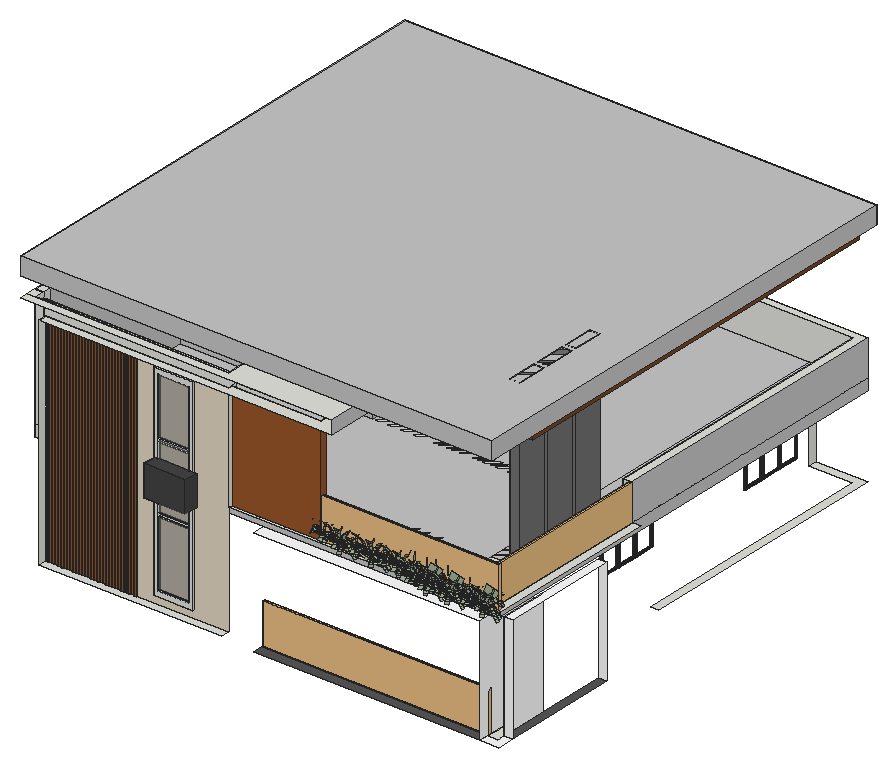
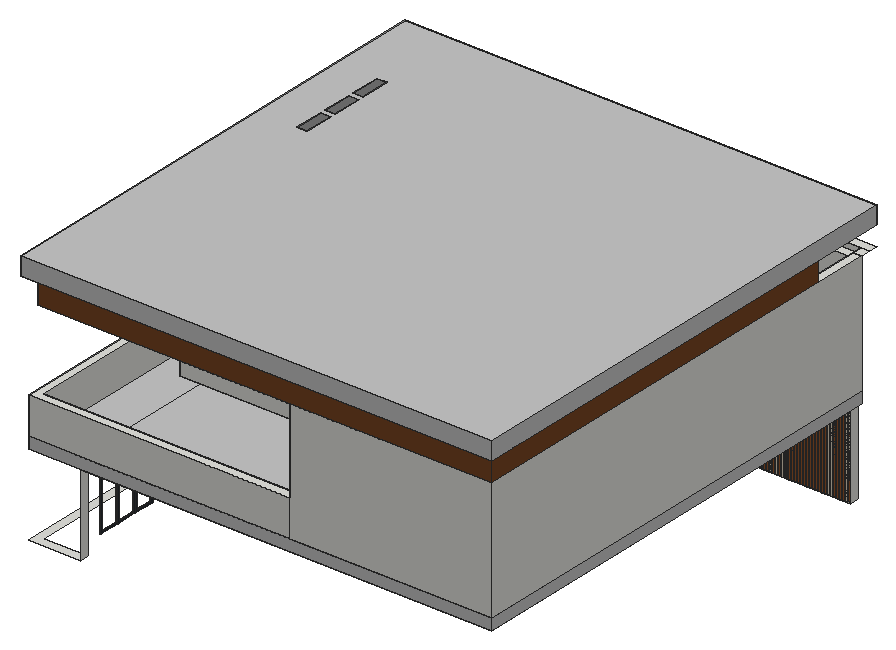
# SketchUp Ruby script. Lengths in inches.
U = 1.inch
M = Sketchup.active_model
def pt(a) = Geom::Point3d.new(a.map { |v| v * U })
def face(e, loops, mat)
  f = e.add_face(loops[0].map { |a| pt(a) })
  loops[1..].each { |l| e.add_face(l.map { |a| pt(a) }).erase! }
  f.material = f.back_material = mat if mat
  f
end
# faces: each face lists its corners as indices into pts; further lists are holes
def faces(e, pts, list, mat = nil) = list.each { |f| face(e, (f[0].is_a?(Array) ? f : [f]).map { |l| l.map { |i| pts[i] } }, mat) }
# xy, xz, yz: faces in a plane at the given z, y or x. An outline is a flat list of corners, or four numbers for a rectangle; further outlines are holes
def ring(l) = l.size == 4 ? [[l[0], l[1]], [l[2], l[1]], [l[2], l[3]], [l[0], l[3]]] : l.each_slice(2).to_a
def flat(e, list, mat, &to3) = list.each { |f| face(e, (f[0].is_a?(Array) ? f : [f]).map { |l| ring(l).map { |u, v| to3.(u, v) } }, mat) }
def xy(e, z, list, mat = nil) = flat(e, list, mat) { |x, y| [x, y, z] }
def xz(e, y, list, mat = nil) = flat(e, list, mat) { |x, z| [x, y, z] }
def yz(e, x, list, mat = nil) = flat(e, list, mat) { |y, z| [x, y, z] }
def lines(e, pts, list) = list.each { |a, b| e.add_line(pt(pts[a]), pt(pts[b])) }
# prism: a flat outline (further loops are holes) pulled along v
def prism(e, loops, v, mat = nil)
  f = face(e, loops, mat); d = Geom::Vector3d.new(v.map { |x| x * U })
  f.pushpull(f.normal.samedirection?(d) ? d.length : -d.length)
end
def box(e, o, s, mat = nil) = prism(e, [[o, [o[0] + s[0], o[1], o[2]], [o[0] + s[0], o[1] + s[1], o[2]], [o[0], o[1] + s[1], o[2]]]], [0, 0, s[2]], mat)
def at(x, y, z, deg = 0) = Geom::Transformation.translation(pt([x, y, z])) * Geom::Transformation.rotation(ORIGIN, Z_AXIS, deg.degrees)
def axes(o, x, y, z) = Geom::Transformation.new([*x, 0, *y, 0, *z, 0, *pt(o).to_a, 1])
def part(name) = M.definitions.add(name)
# library, detail: a bought-in or finely detailed component or shape, given as its bounding box
def library(name, o, s) = part(name).tap { |d| box(d.entities, o, s) }
def detail(e, o, s) = box(e.add_group.entities, o, s)
def put(e, d, t, mat = nil) = e.add_instance(d, t).tap { |i| i.material = mat if mat }
def group(e, t, mat = nil) = e.add_group.tap { |g| g.transformation = t; g.material = mat if mat }.entities
root = M.entities
M.materials.add("Wine2").color = [0, 0, 0]
M.materials["Wine2"].alpha = 0
M.materials.add("[0130_Gainsboro]").color = [39, 45, 50]
M.materials.add("[Color M00]").color = [255, 255, 255]
M.materials.add("[Color M02]").color = [198, 198, 198]
M.materials.add("[Color M05]").color = [114, 114, 114]
M.materials.add("[Color M06]").color = [86, 86, 86]
M.materials.add("[Granite Dark Gray]").color = [69, 68, 68]
M.materials.add("[Stone Brushed Khaki]").color = [226, 216, 194]
M.materials.add("[Translucent Glass Gray]1").color = [128, 128, 128]
M.materials["[Translucent Glass Gray]1"].alpha = 0.5
M.materials.add("[Wood Cherry Original]").color = [152, 86, 42]
M.materials.add("[Wood Veneer 01]").color = [120, 70, 37]
M.materials.add("hymenocallis littoralis").color = [156, 172, 146]
c1 = library("Wagner Glass Railing",[9.08,102.375,1.53],[2.51,145.5,42.05])
c2 = part("Group\#4")
box(c2.entities,[0,0,0],[3,0.5,225.5])
c3 = part("Window")
xy(c3.entities,0,[[0,0,19.69,1.97]])
xy(c3.entities,1.97,[[1.97,0,17.72,0.79]])
xy(c3.entities,1.97,[[1.97,0.79,17.72,1.97]],"[Translucent Glass Gray]1")
xy(c3.entities,24.8,[[1.97,0,17.72,0.79]])
xy(c3.entities,24.8,[[1.97,0.79,17.72,1.97]],"[Translucent Glass Gray]1")
xy(c3.entities,25.98,[[1.97,0,17.72,0.79],[1.97,0.79,17.72,1.97]])
xy(c3.entities,48.03,[[1.97,0,17.72,1.97]])
xy(c3.entities,49.21,[[1.97,0,17.72,0.79]])
xy(c3.entities,49.21,[[1.97,0.79,17.72,1.97]],"[Translucent Glass Gray]1")
xy(c3.entities,68.9,[[1.97,0,17.72,0.79]])
xy(c3.entities,68.9,[[1.97,0.79,17.72,1.97]],"[Translucent Glass Gray]1")
xy(c3.entities,70.87,[[0,0,19.69,1.97]])
xz(c3.entities,0,[[[0,0,19.69,70.87],[1.97,1.97,17.72,68.9]]])
xz(c3.entities,0.79,[[1.97,1.97,17.72,24.8],[1.97,25.98,17.72,48.82],[1.97,49.21,17.72,68.9]],"[Translucent Glass Gray]1")
xz(c3.entities,1.97,[[[0,0,19.69,70.87],[1.97,1.97,17.72,68.9]],[1.97,24.8,17.72,25.98],[1.97,48.03,17.72,49.21]])
yz(c3.entities,0,[[0,0,1.97,70.87]])
yz(c3.entities,1.97,[[0,1.97,0.79,24.8],[0,24.8,1.97,25.98],[0,25.98,0.79,48.03],[0.79,25.98,1.97,48.03],[0,48.03,1.97,49.21],
  [0,49.21,0.79,68.9]])
yz(c3.entities,1.97,[[0.79,1.97,1.97,24.8],[0.79,49.21,1.97,68.9]],"[Translucent Glass Gray]1")
yz(c3.entities,17.72,[[0,1.97,0.79,24.8],[0,24.8,1.97,25.98],[0,25.98,0.79,48.03],[0.79,25.98,1.97,48.03],[0,48.03,1.97,49.21],
  [0,49.21,0.79,68.9]])
yz(c3.entities,17.72,[[0.79,1.97,1.97,24.8],[0.79,49.21,1.97,68.9]],"[Translucent Glass Gray]1")
yz(c3.entities,19.69,[[0,0,1.97,70.87]])
c4 = part("Facade screen panel")
xy(c4.entities,0,[[0,-0.98,43.07,0],[0,0,43.07,1.4]],"[0130_Gainsboro]")
xy(c4.entities,0.3,[[0.3,-1.43,42.77,-0.98]],"[0130_Gainsboro]")
xy(c4.entities,2.95,[[2.95,-1.43,40.12,-0.63],[2.95,-0.63,40.12,0],[2.95,0,40.12,0.64],[2.95,0.64,40.12,1.4]],"[0130_Gainsboro]")
xy(c4.entities,3.54,[[3.54,-0.63,39.53,0],[3.54,0,39.53,0.64]],"[0130_Gainsboro]")
xy(c4.entities,111.8125,[[3.54,-0.63,39.53,0],[3.54,0,39.53,0.64]],"[0130_Gainsboro]")
xy(c4.entities,112.4,[[2.95,-1.43,40.12,-0.63],[2.95,-0.63,40.12,0],[2.95,0,40.12,0.64],[2.95,0.64,40.12,1.4]],"[0130_Gainsboro]")
xy(c4.entities,115.05,[[0.3,-1.43,42.77,-0.98]],"[0130_Gainsboro]")
xy(c4.entities,115.35,[[0,-0.98,43.07,0],[0,0,43.07,1.4]],"[0130_Gainsboro]")
xz(c4.entities,-1.43,[[[0.3,0.3,42.77,115.05],[2.95,2.95,40.12,112.4]]],"[0130_Gainsboro]")
xz(c4.entities,-0.98,[[[0,0,43.07,115.35],[0.3,0.3,42.77,115.05]]],"[0130_Gainsboro]")
xz(c4.entities,-0.63,[[[2.95,2.95,40.12,112.4],[3.54,3.54,39.53,111.8125]]],"[0130_Gainsboro]")
xz(c4.entities,0,[[3.54,3.54,39.53,111.8125]],"Wine2")
xz(c4.entities,0,[[[0,0,43.07,115.35],[2.95,2.95,40.12,112.4]],[[2.95,2.95,40.12,112.4],[3.54,3.54,39.53,111.8125]]],"[0130_Gainsboro]")
xz(c4.entities,0.64,[[[2.95,2.95,40.12,112.4],[3.54,3.54,39.53,111.8125]]],"[0130_Gainsboro]")
xz(c4.entities,1.4,[[[0,0,43.07,115.35],[2.95,2.95,40.12,112.4]]],"[0130_Gainsboro]")
yz(c4.entities,0,[[-0.98,0,0,115.35],[0,0,1.4,115.35]],"[0130_Gainsboro]")
yz(c4.entities,0.3,[[-1.43,0.3,-0.98,115.05]],"[0130_Gainsboro]")
yz(c4.entities,2.95,[[-1.43,2.95,-0.63,112.4],[-0.63,2.95,0,112.4],[0,2.95,0.64,112.4],[0.64,2.95,1.4,112.4]],"[0130_Gainsboro]")
yz(c4.entities,3.54,[[-0.63,3.54,0,111.8125],[0,3.54,0.64,111.8125]],"[0130_Gainsboro]")
yz(c4.entities,39.53,[[-0.63,3.54,0,111.8125],[0,3.54,0.64,111.8125]],"[0130_Gainsboro]")
yz(c4.entities,40.12,[[-1.43,2.95,-0.63,112.4],[-0.63,2.95,0,112.4],[0,2.95,0.64,112.4],[0.64,2.95,1.4,112.4]],"[0130_Gainsboro]")
yz(c4.entities,42.77,[[-1.43,0.3,-0.98,115.05]],"[0130_Gainsboro]")
yz(c4.entities,43.07,[[-0.98,0,0,115.35],[0,0,1.4,115.35]],"[0130_Gainsboro]")
c5 = part("Facade screen assembly")
put(c5.entities,c4,axes([90.57,1.43,0],[1.05148,0,0],[0,1,0],[0,0,1]))
put(c5.entities,c4,axes([0,1.43,0],[1.05148,0,0],[0,1,0],[0,0,1]))
put(c5.entities,c4,axes([45.29,1.43,0],[1.05148,0,0],[0,1,0],[0,0,1]))
c6 = part("Group\#1")
prism(c6.entities,[[[0,0,12],[425.4375,0,12],[480,0,12],[480,0,0],[0,0,0]]],[0,-480,0])
c7 = part("Group\#856")
xy(c7.entities,7.38,[[0,0,5.5,15.91]],"hymenocallis littoralis")
p = [[5.5,28.78,0],[5.5,26.79,3.44],[0,26.79,3.44],[0,28.78,0],[0,23.75,6],[5.5,23.75,6],
  [0,15.91,7.38],[5.5,15.91,7.38]]
faces(c7.entities,p,[[0,1,2,3],[4,2,1,5],[6,4,5,7]],"hymenocallis littoralis")
c8 = part("Group\#854")
xy(c8.entities,7.38,[[0,0,5.5,15.91],[0,15.91,5.5,23.87]],"hymenocallis littoralis")
p = [[5.5,31.07,4.3],[5.5,27.74,6.47],[0,27.74,6.47],[0,31.07,4.3],[0,23.87,7.38],[5.5,23.87,7.38]]
faces(c8.entities,p,[[0,1,2,3],[4,2,1,5]],"hymenocallis littoralis")
c9 = part("Group\#857")
xy(c9.entities,7.38,[[0,0,5.6,15.91]],"hymenocallis littoralis")
p = [[5.6,28.78,0],[5.6,26.79,3.44],[0,26.79,3.44],[0,28.78,0],[0,23.75,6],[5.6,23.75,6],
  [0,15.91,7.38],[5.6,15.91,7.38]]
faces(c9.entities,p,[[0,1,2,3],[4,2,1,5],[6,4,5,7]],"hymenocallis littoralis")
c10 = part("Group\#855")
put(c10.entities,c8,axes([6.09,8.57,-0.52],[0.446,0.85617,0.26089],[-0.18444,-0.19731,0.96283],[0.87582,-0.47754,0.0699]))
put(c10.entities,c8,axes([6.29,7.28,-1.71],[0.37058,0.92707,-0.05667],[-0.32382,0.19004,0.99128],[0.87712,-0.32925,0.34964]))
put(c10.entities,c8,axes([11.04,16.14,-0.7],[1,0,0],[0,0.16628,1.02662],[0,-1.18456,0.19186]))
c11 = part("Group\#860")
put(c11.entities,c7,axes([24.57,32.05,-1.76],[0.9552,-0.22102,-0.19681],[0.4036,0.95545,0.88585],[-0.00568,-0.67859,0.7345]))
put(c11.entities,c7,axes([23.95,29.24,-2.4],[0,1,0],[-0.76041,0,0.64945],[0.64945,0,0.76041]))
put(c11.entities,c7,axes([24.22,24.72,-0.48],[-0.70711,0.70711,0],[-0.32757,-0.32757,0.80237],[0.61237,0.61237,0.5]))
put(c11.entities,c8,axes([20.66,37.22,-0.63],[1.12361,0.03262,0.39091],[-0.43499,0.29739,0.78777],[0.09852,-1.27434,0.37535]))
put(c11.entities,c7,axes([28.75,24.45,-2.4],[-1,0,0],[0,-0.76041,0.64945],[0,0.64945,0.76041]))
put(c11.entities,c9,axes([30.4,30.98,-3.7],[0.65676,-0.72002,0.22414],[0.55667,0.66341,0.5],[-0.50871,-0.20361,0.83652]))
put(c11.entities,c9,axes([32.41,29.61,-3.7],[0.04029,-0.97372,0.22414],[0.85287,0.15038,0.5],[-0.52057,0.17102,0.83652]))
put(c11.entities,c7,axes([31.89,25.85,-1.76],[-0.92056,0.33739,-0.19681],[-0.5186,-0.89824,0.88585],[0.08952,0.67268,0.7345]))
put(c11.entities,c7,axes([25.55,34.78,-0.48],[0.86603,0.5,0],[-0.25,0.43301,0.86603],[0.43301,-0.75,0.5]))
put(c11.entities,c9,axes([20.4,16.9375,-8.07],[-0.70711,0.70711,0],[-0.35754,-0.35754,0.65422],[1.3987,1.3987,1.52882]))
put(c11.entities,c7,axes([32.86,34.14,-0.48],[0.76604,-0.64279,0],[0.32139,0.38302,0.86603],[-0.55667,-0.66341,0.5]))
put(c11.entities,c7,axes([27.15,34.7,-0.1],[0.82472,-0.17528,-0.53769],[0.53769,0.53769,0.64945],[0.17528,-0.82472,0.53769]))
put(c11.entities,c7,axes([33.58,28.77,-2.4],[0,-1,0],[0.76041,0,0.64945],[-0.64945,0,0.76041]))
put(c11.entities,c7,axes([26.43,23.87,-2.81],[-0.75126,0.04415,0.65853],[0.53769,-0.53769,0.64945],[0.38276,0.84199,0.3802]))
put(c11.entities,c7,axes([28.78,23.98,-2.4],[-1,0,0],[0,-0.76041,0.64945],[0,0.64945,0.76041]))
put(c11.entities,c7,axes([25.39,25.38,-2.4],[-0.70711,0.70711,0],[-0.53769,-0.53769,0.64945],[0.45923,0.45923,0.76041]))
put(c11.entities,c7,axes([27.32,21.63,-0.1],[-0.45923,0.70711,-0.53769],[-0.76041,0,0.64945],[0.45923,0.70711,0.53769]))
put(c11.entities,c7,axes([25.17,27.625,-1.76],[0.56416,0.80187,-0.19681],[-0.66673,0.66673,0.80532],[0.62659,-0.26057,0.7345]))
put(c11.entities,c9,axes([27.59,27.04,-3.96],[-0.8993,-0.06127,0.43301],[0.2962,-0.8138,0.5],[0.32175,0.57791,0.75]))
put(c11.entities,c9,axes([26.98,24.5,-3.18],[-0.5,0.86603,0],[-0.75,-0.43301,0.5],[0.43301,0.25,0.86603]))
put(c11.entities,c9,axes([24.55,27.74,-3.7],[0.29517,0.92878,0.22414],[-0.85287,0.15038,0.5],[0.43068,-0.33875,0.83652]))
put(c11.entities,c9,axes([24.26,29.8,-3.18],[0.76604,0.64279,0],[-0.47317,0.5639,0.425],[0.32139,-0.38302,0.86603]))
put(c11.entities,c9,axes([25.98,32.46,-3.18],[1,0,0],[0,0.86603,0.5],[0,-0.5,0.86603]))
put(c11.entities,c7,axes([28.78,33.57,-2.4],[1,0,0],[0,0.76041,0.64945],[0,-0.64945,0.76041]))
put(c11.entities,c10,at(14.99,21.38,2.5))
put(c11.entities,c8,axes([34.63,26.34,-1.46],[-0.70089,-0.70877,0.07994],[0.4756,-0.38088,0.79293],[-0.53156,0.59378,0.60405]))
put(c11.entities,c8,axes([28.14,16.92,1.8125],[-1.19719,0.6912,0],[-0.09607,-0.16641,0.94244],[0.68444,1.18549,0.17613]))
put(c11.entities,c8,axes([31.5625,35.84,0.97],[0.66765,-1.1564,0.35779],[0.04445,0.30732,0.91033],[-1.20828,-0.64496,0.17012]))
put(c11.entities,c8,axes([38.94,22.51,0.89],[-0.97932,-0.67164,-0.05202],[0.27787,-0.41401,0.90999],[-0.85985,0.93577,0.32097]))
put(c11.entities,c8,axes([38.44,21.09,1.98],[-1.02864,-0.54856,0.2395],[0.33481,0.06999,0.88388],[-0.77261,1.08328,0.06417]))
put(c11.entities,c9,axes([35.02,30.51,-1.3],[-0.17365,-0.98481,0],[0.60224,-0.10619,0.79122],[-0.7792,0.13739,0.61153]))
put(c11.entities,c9,axes([29.41,22.33,-1.3],[-0.93969,0.34202,0],[-0.20915,-0.57465,0.79122],[0.27061,0.74351,0.61153]))
put(c11.entities,c8,axes([19.64,36,-1.62],[1.18194,0.09546,0.08234],[-0.14377,0.68823,0.76313],[0.21457,-1.1326,0.62386]))
put(c11.entities,c9,axes([24.25,24.14,-1.3],[-0.34202,0.93969,0],[-0.57465,-0.20915,0.79122],[0.74351,0.27061,0.61153]))
put(c11.entities,c9,axes([25.98,34.61,-1.3],[1,0,0],[0,0.61153,0.79122],[0,-0.79122,0.61153]))
put(c11.entities,c9,axes([31.16,34.41,-1.64],[0.56518,-0.80224,-0.19234],[0.73413,0.34233,0.72935],[-0.47639,-0.50772,0.71782]))
put(c11.entities,c9,axes([40.52,26.84,-5.82],[-0.42262,-0.90631,0],[0.48019,-0.22391,0.68552],[-1.43418,0.66877,1.22305]))
put(c11.entities,c7,axes([29.86,38.42,-1.01],[0.89064,-0.37013,0.26413],[-0.03924,0.63286,1.01918],[-0.45353,-0.76487,0.45748]))
put(c11.entities,c7,axes([29.34,22.4,-0.48],[-0.99619,-0.08716,0],[0.04358,-0.4981,0.86603],[-0.07548,0.86273,0.5]))
c12 = part("Group\#858")
xz(c12.entities,10.07,[[9.07,0,10.07,31.01],[0,31.01,0,45.12,20.13,45.12,20.13,31.01,10.07,31.01,10.07,32.58,9.07,32.58,9.07,31.01]],"hymenocallis littoralis")
yz(c12.entities,10.07,[[0,31.01,20.13,45.12]],"hymenocallis littoralis")
p = [[9.57,9.2,0],[10.07,10.07,0],[10.07,10.07,31.01],[10.07,10.07,32.58],[9.57,9.2,32.58]]
faces(c12.entities,p,[[0,1,2,3,4]],"hymenocallis littoralis")
c13 = part("cây lá nắng")
put(c13.entities,c11,axes([49.26,-2.75,0],[0.63109,0.63109,0],[-0.63109,0.63109,0],[0,0,0.935]))
g1 = group(c13.entities,at(26.6,-8.68,0))
put(g1,c7,axes([-4.72,35.73,-1.65],[0.74231,0.46334,-0.18402],[-0.34827,0.85768,0.82827],[0.42467,-0.43184,0.68675]))
put(g1,c7,axes([-3.34,33.57,-2.24],[-0.63109,0.63109,0],[-0.47989,-0.47989,0.60723],[0.40986,0.40986,0.71098]))
put(g1,c7,axes([-0.3125,30.89,-0.45],[-0.8925,0,0],[0,-0.41345,0.75022],[0,0.77293,0.4675]))
put(g1,c8,axes([-10.79,39.66,-0.59],[0.68852,0.72969,0.3655],[-0.4622,-0.08684,0.73657],[0.86641,-0.74205,0.35095]))
put(g1,c7,axes([2.71,33.57,-2.24],[-0.63109,-0.63109,0],[0.47989,-0.47989,0.60723],[-0.40986,0.40986,0.71098]))
put(g1,c9,axes([-0.37,38.74,-3.46],[0.86887,-0.03992,0.20957],[-0.06737,0.76999,0.4675],[-0.19255,-0.44954,0.78214]))
put(g1,c9,axes([1.76,39.14,-3.46],[0.63993,-0.58908,0.20957],[0.44333,0.63315,0.4675],[-0.43646,-0.2206,0.78214]))
put(g1,c7,axes([3.81,36.4375,-1.65],[-0.79389,-0.36803,-0.18402],[0.23959,-0.89415,0.82827],[-0.36803,0.48102,0.68675]))
put(g1,c7,axes([-5.83,38.07,-0.45],[0.231,0.86209,0],[-0.43104,0.1155,0.80973],[0.74659,-0.20005,0.4675]))
put(g1,c9,axes([2.18,23.5625,-7.55],[-0.8925,0,0],[0,-0.45128,0.6117],[0,1.76542,1.42944]))
put(g1,c7,axes([-0.8125,42.28,-0.45],[0.8891,0.07779,0],[-0.03889,0.44455,0.80973],[0.06737,-0.76999,0.4675]))
put(g1,c7,axes([-4.76,39.03,-0.09],[0.63109,0.40986,-0.50274],[0,0.67866,0.60723],[0.63109,-0.40986,0.50274]))
put(g1,c7,axes([3.03,39.35,-2.24],[0.63109,-0.63109,0],[0.47989,0.47989,0.60723],[-0.40986,-0.40986,0.71098]))
put(g1,c7,axes([1.61,31.74,-2.625],[-0.50198,-0.44625,0.61573],[0.67866,0,0.60723],[-0.28982,0.77293,0.35549]))
put(g1,c7,axes([3.03,33.3,-2.24],[-0.63109,-0.63109,0],[0.47989,-0.47989,0.60723],[-0.40986,0.40986,0.71098]))
put(g1,c7,axes([0.01,32.04,-2.24],[-0.8925,0,0],[0,-0.67866,0.60723],[0,0.57963,0.71098]))
put(g1,c7,axes([3.59,30.89,-0.09],[-0.73607,0.15643,-0.50274],[-0.47989,-0.47989,0.60723],[-0.15643,0.73607,0.50274]))
put(g1,c7,axes([-1.55,33.32,-1.65],[-0.15002,0.86209,-0.18402],[-0.84154,0,0.75297],[0.55988,0.231,0.68675]))
put(g1,c9,axes([0.35,34.48,-3.71],[-0.52887,-0.60621,0.40487],[0.70051,-0.32665,0.4675],[-0.16166,0.56777,0.70125]))
put(g1,c9,axes([2.61,39.13,-1.74],[-0.86209,0.231,0],[-0.23031,-0.85954,0.15531],[0.03162,0.11799,0.91645]))
put(g1,c9,axes([-2.02,33,-3.46],[-0.39986,0.77243,0.20957],[-0.63315,-0.44333,0.4675],[0.48558,0.05802,0.78214]))
put(g1,c9,axes([-3.49,34.12,-2.97],[0.07779,0.8891,0],[-0.65449,0.05726,0.39737],[0.44455,-0.03889,0.80973]))
put(g1,c9,axes([-4.09,36.88,-2.97],[0.63109,0.63109,0],[-0.54654,0.54654,0.4675],[0.31555,-0.31555,0.80973]))
put(g1,c7,axes([-3.02,39.35,-2.24],[0.63109,0.63109,0],[-0.47989,0.47989,0.60723],[0.40986,-0.40986,0.71098]))
put(g1,c10,axes([-4.03,22.95,2.33],[0.63109,0.63109,0],[-0.63109,0.63109,0],[0,0,0.935]))
put(g1,c8,axes([5.24,38.48,-1.37],[0.00497,-0.88963,0.07474],[0.54052,0.05978,0.74139],[-0.71019,0.03927,0.56479]))
put(g1,c8,axes([7.08,28.4375,1.7],[-1.19175,-0.31933,0],[0.04439,-0.16565,0.88118],[-0.31621,1.1801,0.16468]))
put(g1,c8,axes([-2.7,42.54,0.91],[1.15114,-0.30845,0.33454],[-0.1659,0.22199,0.85115],[-0.3555,-1.16957,0.15907]))
put(g1,c8,axes([10.37,38.78,0.83],[-0.19417,-1.04191,-0.04864],[0.43664,-0.08592,0.85084],[-1.1332,0.04791,0.30011]))
put(g1,c8,axes([10.95,37.5625,1.85],[-0.30298,-0.99536,0.22393],[0.16713,0.25547,0.82643],[-1.17124,0.19607,0.06]))
put(g1,c9,axes([2.84,41.36,-1.22],[0.51192,-0.73109,0],[0.44708,0.31305,0.73979],[-0.57846,-0.40504,0.57178]))
put(g1,c9,axes([4.47,32.65,-1.22],[-0.80888,-0.37719,0],[0.23066,-0.49465,0.73979],[-0.29844,0.64,0.57178]))
put(g1,c8,axes([-10.32,35.12,-1.51],[0.68567,0.80616,0.07699],[-0.52507,0.3436,0.71352],[0.85019,-0.57936,0.58331]))
put(g1,c9,axes([0.07,30.54,-1.22],[-0.80888,0.37719,0],[-0.23066,-0.49465,0.73979],[0.29844,0.64,0.57178]))
put(g1,c9,axes([-5.45,38.24,-1.22],[0.63109,0.63109,0],[-0.38593,0.38593,0.73979],[0.49934,-0.49934,0.57178]))
put(g1,c9,axes([-2.05,41.38,-1.53],[0.86296,-0.14961,-0.17984],[0.24726,0.67935,0.68194],[0.01977,-0.62107,0.67116]))
put(g1,c9,axes([8.63,42.51,-5.4375],[0.30525,-0.83868,0],[0.44435,0.16173,0.64096],[-1.32716,-0.48305,1.14356]))
put(g1,c7,axes([-5.4,43.09,-0.94],[0.79566,0.32849,0.24696],[-0.42416,0.37462,0.95293],[0.19648,-0.76892,0.42774]))
put(g1,c7,axes([4.38,32.65,-0.45],[-0.57369,-0.68369,0],[0.34185,-0.28684,0.80973],[-0.5921,0.49683,0.4675]))
put(g1,c9,axes([-2,33.84,-0.15],[-0.24601,0.85793,0],[-0.85539,-0.24528,0.15531],[0.11742,0.03367,0.91645]))
put(g1,c9,axes([0.17,30.83,-4.47],[-0.24601,0.85793,0],[-0.85539,-0.24528,0.15531],[0.11742,0.03367,0.91645]))
put(g1,c9,axes([-1.97,32.18,-4.47],[0.58524,0.67383,0],[-0.67184,0.58351,0.15531],[0.09222,-0.0801,0.91645]))
put(g1,c9,axes([-2,34.71,-4.47],[0.88392,-0.12346,0],[0.12309,0.88131,0.15531],[-0.0169,-0.12098,0.91645]))
put(g1,c9,axes([0.11,36.12,-4.47],[0.37822,-0.8084,0],[0.80601,0.37711,0.15531],[-0.11064,-0.05177,0.91645]))
put(c13.entities,c12,axes([29.71,14.29,6.94],[0.425,0.73612,0],[-0.6771,0.39092,-0.33349],[-0.26859,0.15507,0.72712]))
put(c13.entities,c12,axes([42.0625,26.12,6.94],[0.85,0,0],[0,0.78185,-0.33349],[0,0.33349,0.78185]))
put(c13.entities,c11,axes([7.3125,23.0625,0],[0.8925,0,0],[0,0.8925,0],[0,0,0.935]))
put(c13.entities,c12,axes([24.4375,40.23,2.05],[0.85,0,0],[0,0.85,0],[0,0,0.85]))
c14 = part("Planting 101")
put(c14.entities,c13,axes([21.34,32.96,-4.59],[0,-0.71,0],[-0.71,0,0],[0,0,0.71]))
c15 = part("Group\#6")
box(c15.entities,[0,0,-164.1875],[10.1875,30.6875,164.1875])
c16 = library("Light 01",[-2.3,-2.42,-0.19],[4.85,4.84,0.19])
xy(root,271.125,[[821.46,131.75,823.1875,190.625],[823.1875,131.75,832.1875,190.625]])
xy(root,271.125,[[821.46,121.8125,840.86,121.8125,840.86,139.96,832.1875,139.96,832.1875,131.75,821.46,131.75]],"[Color M00]")
xy(root,271.125,[[587.02,121.8125,821.46,131.75],[832.1875,139.96,840.86,262.46]],"[Color M06]")
xy(root,280.08,[[371.42,112.8125,561,112.8125,561,121.8125,373.48,121.8125,373.48,121.3125,371.42,121.3125]])
xy(root,299.4375,[[823.1875,340.9375,832.1875,340.9375,832.1875,611.75,777.625,611.75,777.625,602.75,823.1875,602.75]])
xy(root,381.625,[[587.02,121.8125,821.46,190.625],[832.1875,139.96,840.86,262.46]],"[Color M00]")
xy(root,384,[[[352.1875,131.75,361.1875,131.75,361.1875,308.68,777.625,308.68,777.625,611.75,352.1875,611.75],[361.1875,317.68,768.625,602.75]]])
xy(root,387.72,[[531.6,102.34,488.17,103.49,488.55,117.86,531.98,116.71]],"[Granite Dark Gray]")
xy(root,396,[[561,121.8125,561,125.8125,653.75,125.8125,653.75,131.75,561,131.75,561,190.625,832.1875,190.625,832.1875,306.4375,840.86,306.4375,840.86,121.8125],[561,125.8125,653.75,131.75],[[352.1875,131.75,361.1875,131.75,361.1875,308.68,561,308.68,561,611.75,352.1875,611.75],[361.1875,317.68,516.8125,602.75]],[361.1875,131.75,561,140.75],[361.1875,140.75,561,140.75,561,190.625,777.625,190.625,777.625,308.68,361.1875,308.68],
  [777.625,190.625,823.1875,308.68],[823.1875,190.625,832.1875,304.99],[561,308.68,823.1875,317.68],[361.1875,317.68,516.8125,602.75]])
xy(root,419.47,[[531.6,102.34,531.98,116.71,488.55,117.86,488.17,103.49]],"[Granite Dark Gray]")
xy(root,434.05,[[823.1875,304.99,832.1875,304.99,832.1875,611.75,561,611.75,561,602.75,823.1875,602.75]])
xy(root,507.32,[[371.42,112.8125,371.42,121.8125,561,121.8125,561,125.8125,653.75,125.8125,653.75,131.75,561,131.75,561,611.75,674.9375,611.75,674.9375,112.8125]])
xy(root,516,[[361.1875,121.8125,561,131.75]])
xy(root,521.25,[[352.1875,112.8125,674.9375,112.8125,674.9375,611.75,561,611.75,561,121.8125,352.1875,121.8125],[352.1875,121.8125,361.1875,131.75],[[352.1875,131.75,361.1875,131.75,361.1875,308.68,561,308.68,561,611.75,352.1875,611.75],[361.1875,317.68,516.8125,602.75]]])
xz(root,121.8125,[[361.1875,516,561,521.25]])
xz(root,121.8125,[[371.42,280.08,561,507.32]],"[Stone Brushed Khaki]")
xz(root,125.8125,[[561,396,653.75,507.32]],"[Wood Cherry Original]")
xz(root,131.75,[[352.1875,384,361.1875,396],[352.1875,396,361.1875,521.25],[361.1875,396,561,516],[561,396,653.75,507.32]])
xz(root,139.96,[[832.1875,271.125,840.86,381.625]],"[Color M00]")
xz(root,262.46,[[832.1875,271.125,840.86,381.625]],"[Color M00]")
xz(root,304.99,[[823.1875,396,832.1875,434.05]])
xz(root,308.68,[[361.1875,396,561,521.25]],"[Color M02]")
xz(root,317.68,[[361.1875,396,516.8125,521.25]])
xz(root,602.75,[[361.1875,396,516.8125,521.25],[561,396,823.1875,434.05]])
xz(root,611.75,[[352.1875,396,561,521.25],[561,396,832.1875,434.05],[561,507.32,674.9375,521.25]])
yz(root,352.1875,[[131.75,396,611.75,521.25]])
yz(root,361.1875,[[131.75,396,140.75,521.25],[317.68,396,602.75,521.25],[121.8125,516,131.75,521.25]])
yz(root,361.1875,[[140.75,396,308.68,521.25]],"[Color M02]")
yz(root,371.42,[[112.8125,280.08,121.8125,507.32]])
yz(root,516.8125,[[317.68,396,602.75,521.25]])
yz(root,561,[[121.8125,396,125.8125,507.32],[125.8125,396,131.75,507.32],[131.75,507.32,308.68,521.25],[308.68,507.32,611.75,521.25],[121.8125,516,131.75,521.25]])
yz(root,561,[[308.68,396,602.75,396,602.75,434.05,611.75,434.05,611.75,507.32,308.68,507.32]],"[Color M02]")
yz(root,653.75,[[125.8125,396,131.75,507.32]],"[Wood Cherry Original]")
yz(root,674.9375,[[112.8125,507.32,611.75,521.25]],"[Color M02]")
yz(root,777.625,[[602.75,299.4375,611.75,384]])
yz(root,821.46,[[121.8125,271.125,190.625,381.625]],"[Color M00]")
yz(root,823.1875,[[304.99,396,317.68,434.05],[317.68,396,602.75,434.05]])
yz(root,832.1875,[[139.96,271.125,190.625,381.625]],"[Color M00]")
yz(root,832.1875,[[304.99,396,611.75,434.05]],"[Color M02]")
p = [[531.6,102.34,419.47],[488.17,103.49,419.47],[488.17,103.49,387.72],[531.6,102.34,387.72],[531.98,116.71,387.72],[531.98,116.71,419.47],
  [488.55,117.86,419.47],[488.55,117.86,387.72]]
faces(root,p,[[0,1,2,3],[4,5,0,3],[6,7,2,1]],"[Granite Dark Gray]")
faces(root,p,[[6,5,4,7]])
put(root,c1,axes([422.07,145.41,269.58],[0,-1,0],[1.61128,0,0],[0,0,1]))
put(root,c2,at(371.42,121.3125,280.08),"[Wood Cherry Original]")
put(root,c2,at(374.6,121.3125,280.08),"[Wood Cherry Original]")
put(root,c2,at(377.79,121.3125,280.08),"[Wood Cherry Original]")
put(root,c2,at(380.98,121.3125,280.08),"[Wood Cherry Original]")
put(root,c2,at(384.17,121.3125,280.08),"[Wood Cherry Original]")
put(root,c2,at(387.35,121.3125,280.08),"[Wood Cherry Original]")
put(root,c2,at(390.48,121.3125,280.08),"[Wood Cherry Original]")
put(root,c2,at(393.6,121.3125,280.08),"[Wood Cherry Original]")
put(root,c2,at(396.73,121.3125,280.08),"[Wood Cherry Original]")
put(root,c2,at(399.79,121.3125,280.08),"[Wood Cherry Original]")
put(root,c2,at(402.92,121.3125,280.08),"[Wood Cherry Original]")
put(root,c2,at(406.04,121.3125,280.08),"[Wood Cherry Original]")
put(root,c2,at(409.17,121.3125,280.08),"[Wood Cherry Original]")
put(root,c2,at(412.22,121.3125,280.08),"[Wood Cherry Original]")
put(root,c2,at(415.35,121.3125,280.08),"[Wood Cherry Original]")
put(root,c2,at(418.47,121.3125,280.08),"[Wood Cherry Original]")
put(root,c2,at(421.54,121.3125,280.08),"[Wood Cherry Original]")
put(root,c2,at(424.66,121.3125,280.08),"[Wood Cherry Original]")
put(root,c2,at(427.79,121.3125,280.08),"[Wood Cherry Original]")
put(root,c2,at(430.97,121.3125,280.08),"[Wood Cherry Original]")
put(root,c2,at(434.16,121.3125,280.08),"[Wood Cherry Original]")
put(root,c2,at(437.35,121.3125,280.08),"[Wood Cherry Original]")
put(root,c2,at(440.54,121.3125,280.08),"[Wood Cherry Original]")
put(root,c2,at(443.79,121.3125,280.08),"[Wood Cherry Original]")
put(root,c2,at(446.97,121.3125,280.08),"[Wood Cherry Original]")
put(root,c2,at(450.1,121.3125,280.08),"[Wood Cherry Original]")
put(root,c2,at(453.35,121.3125,280.08),"[Wood Cherry Original]")
put(root,c2,at(456.66,121.3125,280.08),"[Wood Cherry Original]")
put(root,c2,at(459.97,121.3125,280.08),"[Wood Cherry Original]")
put(root,c2,at(463.29,121.3125,280.08),"[Wood Cherry Original]")
put(root,c3,axes([487.625,116.9375,290.67],[2.0276,0,0],[0,1,0],[0,0,3]))
put(root,c5,axes([778.33,333.41,313.29],[0,0.4896,0],[-0.4896,0,0],[0,0,0.4896]))
put(root,c5,axes([778.33,520.47,313.29],[0,0.4896,0],[-0.4896,0,0],[0,0,0.4896]))
put(root,c6,at(352.1875,611.75,384),"[Color M02]")
put(root,c14,axes([810.8,123.38,394.29],[0,-0.53939,0],[1,0,0],[0,0,1]))
put(root,c14,axes([753.71,121.93,394.74],[0,-0.53939,0],[1,0,0],[0,0,1]))
put(root,c14,axes([775.84,121.93,394.74],[0,-0.53939,0],[1,0,0],[0,0,1]))
put(root,c14,axes([659.97,127.08,397.84],[0,-0.53939,0],[1,0,0],[0,0,1]))
put(root,c14,axes([692.97,127.08,397.84],[0,-0.53939,0],[1,0,0],[0,0,1]))
put(root,c14,axes([721.47,127.08,397.84],[0,-0.53939,0],[1,0,0],[0,0,1]))
put(root,c1,axes([820.6,9.52,394.625],[1,0,0],[0,1.19199,0],[0,0,0.897]))
put(root,c15,at(788.61,202.05,560.1875),"[Color M05]")
put(root,c15,at(788.61,238.37,560.1875),"[Color M05]")
put(root,c15,at(788.61,274.68,560.1875),"[Color M05]")
put(root,c1,axes([523.72,137.41,394.47],[0,-1,0],[1.2701,0,0],[0,0,1]))
put(root,c16,axes([659.01,197.88,507.32],[3.32,0,0],[0,3.32,0],[0,0,3.32]))
g2 = group(root,at(352.1875,611.75,521.25),"[Color M02]")
xy(g2,0,[[[0,-423.3125,471,0],[17.47,-405.84,453.53,-17.47]]])
xy(g2,20.3125,[[0,-498.9375,488.67,-423.3125],[[0,-423.3125,471,0],[17.47,-405.84,453.53,-17.47]],[471,-423.3125,488.67,0]])
xy(g2,38.9375,[[0,-498.9375,488.67,0]])
xz(g2,-498.9375,[[0,20.3125,488.67,38.9375]])
xz(g2,-423.3125,[[0,0,471,20.3125]],"[Wood Veneer 01]")
xz(g2,-405.84,[[17.47,0,453.53,20.3125]])
xz(g2,-17.47,[[17.47,0,453.53,20.3125]])
xz(g2,0,[[0,20.3125,488.67,38.9375]])
xz(g2,0,[[0,0,471,20.3125]],"[Wood Veneer 01]")
yz(g2,0,[[-498.9375,20.3125,0,38.9375]])
yz(g2,0,[[-423.3125,0,0,20.3125]],"[Wood Veneer 01]")
yz(g2,17.47,[[-405.84,0,-17.47,20.3125]])
yz(g2,453.53,[[-405.84,0,-17.47,20.3125]])
yz(g2,471,[[-423.3125,0,0,20.3125]],"[Wood Veneer 01]")
yz(g2,488.67,[[-498.9375,20.3125,0,38.9375]])
put(root,c16,axes([720.78,128.32,541.5625],[3.32,0,0],[0,3.32,0],[0,0,3.32]))
put(root,c16,axes([609.84,128.32,541.5625],[3.32,0,0],[0,3.32,0],[0,0,3.32]))
put(root,c16,axes([826.78,128.32,541.5625],[3.32,0,0],[0,3.32,0],[0,0,3.32]))
put(root,c16,axes([503.78,128.32,541.5625],[3.32,0,0],[0,3.32,0],[0,0,3.32]))
put(root,c16,axes([371.22,128.32,541.5625],[3.32,0,0],[0,3.32,0],[0,0,3.32]))
